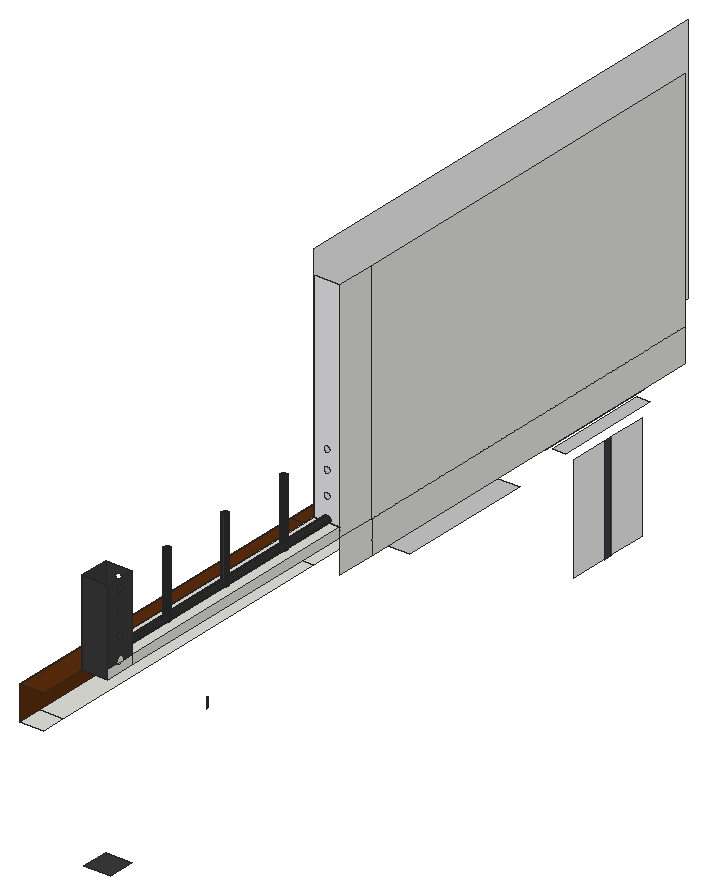
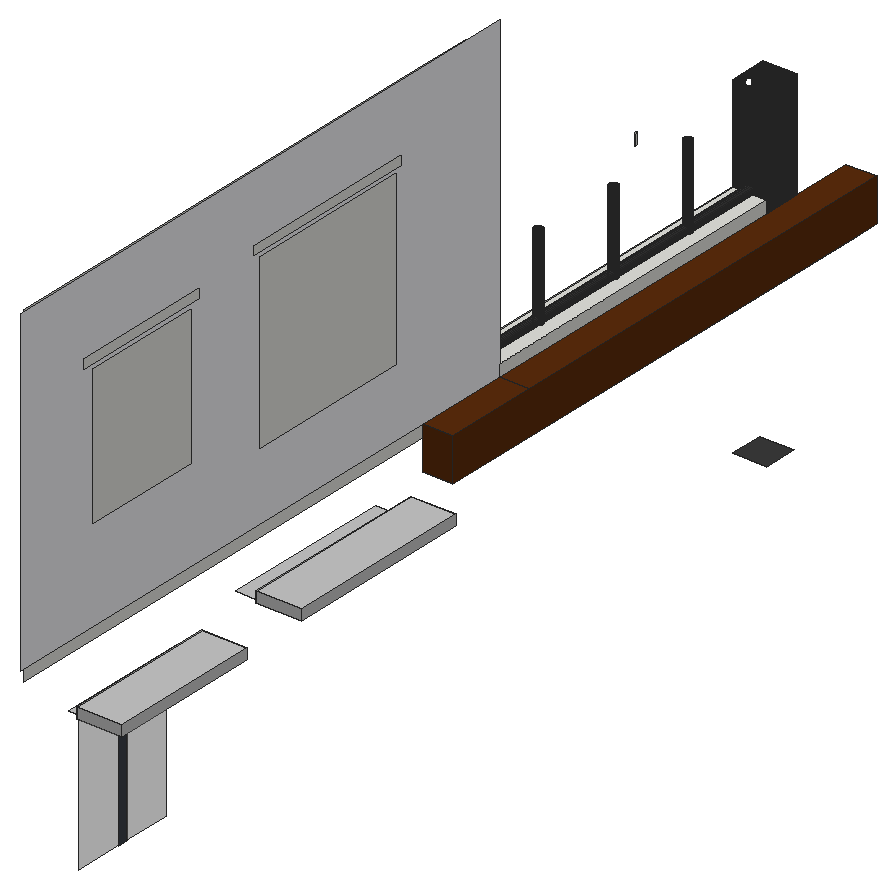
# SketchUp Ruby script. Lengths in inches.
U = 1.inch
M = Sketchup.active_model
def pt(a) = Geom::Point3d.new(a.map { |v| v * U })
def face(e, loops, mat)
  f = e.add_face(loops[0].map { |a| pt(a) })
  loops[1..].each { |l| e.add_face(l.map { |a| pt(a) }).erase! }
  f.material = f.back_material = mat if mat
  f
end
# faces: each face lists its corners as indices into pts; further lists are holes
def faces(e, pts, list, mat = nil) = list.each { |f| face(e, (f[0].is_a?(Array) ? f : [f]).map { |l| l.map { |i| pts[i] } }, mat) }
# xy, xz, yz: faces in a plane at the given z, y or x. An outline is a flat list of corners, or four numbers for a rectangle; further outlines are holes
def ring(l) = l.size == 4 ? [[l[0], l[1]], [l[2], l[1]], [l[2], l[3]], [l[0], l[3]]] : l.each_slice(2).to_a
def flat(e, list, mat, &to3) = list.each { |f| face(e, (f[0].is_a?(Array) ? f : [f]).map { |l| ring(l).map { |u, v| to3.(u, v) } }, mat) }
def xy(e, z, list, mat = nil) = flat(e, list, mat) { |x, y| [x, y, z] }
def xz(e, y, list, mat = nil) = flat(e, list, mat) { |x, z| [x, y, z] }
def yz(e, x, list, mat = nil) = flat(e, list, mat) { |y, z| [x, y, z] }
def lines(e, pts, list) = list.each { |a, b| e.add_line(pt(pts[a]), pt(pts[b])) }
# prism: a flat outline (further loops are holes) pulled along v
def prism(e, loops, v, mat = nil)
  f = face(e, loops, mat); d = Geom::Vector3d.new(v.map { |x| x * U })
  f.pushpull(f.normal.samedirection?(d) ? d.length : -d.length)
end
def box(e, o, s, mat = nil) = prism(e, [[o, [o[0] + s[0], o[1], o[2]], [o[0] + s[0], o[1] + s[1], o[2]], [o[0], o[1] + s[1], o[2]]]], [0, 0, s[2]], mat)
def at(x, y, z, deg = 0) = Geom::Transformation.translation(pt([x, y, z])) * Geom::Transformation.rotation(ORIGIN, Z_AXIS, deg.degrees)
def axes(o, x, y, z) = Geom::Transformation.new([*x, 0, *y, 0, *z, 0, *pt(o).to_a, 1])
def part(name) = M.definitions.add(name)
# library, detail: a bought-in or finely detailed component or shape, given as its bounding box
def library(name, o, s) = part(name).tap { |d| box(d.entities, o, s) }
def detail(e, o, s) = box(e.add_group.entities, o, s)
def put(e, d, t, mat = nil) = e.add_instance(d, t).tap { |i| i.material = mat if mat }
def group(e, t, mat = nil) = e.add_group.tap { |g| g.transformation = t; g.material = mat if mat }.entities
root = M.entities
M.materials.add("[0043_SaddleBrown]").color = [91, 44, 12]
M.materials.add("[Blinds Vertical Pattern]").color = [237, 237, 239]
M.materials.add("[Color M02]").color = [198, 198, 198]
M.materials.add("[Color M07]").color = [58, 58, 58]
M.materials.add("[Formica Laminate Dark]").color = [59, 63, 71]
M.materials.add("[Translucent Glass Gray]").color = [128, 128, 128]
M.materials["[Translucent Glass Gray]"].alpha = 0.5
xy(root,315.4375,[[73.92,405.6875,85.98,418.04]],"[Color M07]")
xy(root,369.09,[[73.92,675.92,79.92,724.73]],"[Color M02]")
xy(root,370.21,[[57.67,672.04,73.92,728.61]],"[Color M02]")
xy(root,370.85,[[73.92,581.05,84.11,644.17]],"[Color M02]")
xy(root,372.15,[[57.67,578.07,73.92,647.71]],"[Color M02]")
xy(root,374.09,[[57.67,672.04,73.92,728.61]],"[Color M02]")
xy(root,376.02,[[57.67,578.07,73.92,647.71]],"[Color M02]")
xy(root,381.625,[[63.07,382.09,73.92,393.34],[63.07,393.34,73.92,538.2],[63.07,538.2,73.92,572.7]])
xy(root,397.0625,[[73.92,404.34,85.98,418.04],[[73.92,418.04,85.98,538.2],[79.95,511.66,80.34,511.71,80.7,511.86,81.01,512.1,81.25,512.41,81.4,512.77,81.45,513.16,81.4,513.55,81.25,513.91,81.01,514.22,80.7,514.46,80.34,514.61,79.95,514.66,79.5625,514.61,79.2,514.46,78.89,514.22,78.65,513.91,78.5,513.55,78.45,513.16,78.5,512.77,78.65,512.41,78.89,512.1,79.2,511.86,79.5625,511.71],[79.95,444.41,80.34,444.46,80.7,444.61,81.01,444.85,81.25,445.16,81.4,445.52,81.45,445.91,81.4,446.3,81.25,446.66,81.01,446.97,80.7,447.21,80.34,447.36,79.95,447.41,79.5625,447.36,79.2,447.21,78.89,446.97,78.65,446.66,78.5,446.3,78.45,445.91,78.5,445.52,78.65,445.16,78.89,444.85,79.2,444.61,79.5625,444.46],[79.95,477.84,80.34,477.9,80.7,478.05,81.01,478.28,81.25,478.59,81.4,478.96,81.45,479.34,81.4,479.73,81.25,480.09,81.01,480.41,80.7,480.64,80.34,480.79,79.95,480.84,79.5625,480.79,79.2,480.64,78.89,480.41,78.65,480.09,78.5,479.73,78.45,479.34,78.5,478.96,78.65,478.59,78.89,478.28,79.2,478.05,79.5625,477.9]],[79.95,444.41,79.5625,444.46,79.2,444.61,78.89,444.85,78.65,445.16,78.5,445.52,78.45,445.91,78.5,446.3,78.65,446.66,78.89,446.97,79.2,447.21,79.5625,447.36,79.95,447.41,80.34,447.36,80.7,447.21,81.01,446.97,81.25,446.66,81.4,446.3,81.45,445.91,81.4,445.52,81.25,445.16,81.01,444.85,80.7,444.61,80.34,444.46],[79.95,477.84,79.5625,477.9,79.2,478.05,78.89,478.28,78.65,478.59,78.5,478.96,78.45,479.34,78.5,479.73,78.65,480.09,78.89,480.41,79.2,480.64,79.5625,480.79,79.95,480.84,80.34,480.79,80.7,480.64,81.01,480.41,81.25,480.09,81.4,479.73,81.45,479.34,81.4,478.96,81.25,478.59,81.01,478.28,80.7,478.05,80.34,477.9],[79.95,511.66,79.5625,511.71,79.2,511.86,78.89,512.1,78.65,512.41,78.5,512.77,78.45,513.16,78.5,513.55,78.65,513.91,78.89,514.22,79.2,514.46,79.5625,514.61,79.95,514.66,80.34,514.61,80.7,514.46,81.01,514.22,81.25,513.91,81.4,513.55,81.45,513.16,81.4,512.77,81.25,512.41,81.01,512.1,80.7,511.86,80.34,511.71]])
xy(root,397.0625,[[63.07,382.09,73.92,538.2],[63.07,538.2,73.92,572.7]],"[0043_SaddleBrown]")
xy(root,401.4375,[[[73.92,418.04,85.98,538.2],[79.95,511.66,79.5625,511.71,79.2,511.86,78.89,512.1,78.65,512.41,78.5,512.77,78.45,513.16,78.5,513.55,78.65,513.91,78.89,514.22,79.2,514.46,79.5625,514.61,79.95,514.66,80.34,514.61,80.7,514.46,81.01,514.22,81.25,513.91,81.4,513.55,81.45,513.16,81.4,512.77,81.25,512.41,81.01,512.1,80.7,511.86,80.34,511.71],[79.95,444.41,79.5625,444.46,79.2,444.61,78.89,444.85,78.65,445.16,78.5,445.52,78.45,445.91,78.5,446.3,78.65,446.66,78.89,446.97,79.2,447.21,79.5625,447.36,79.95,447.41,80.34,447.36,80.7,447.21,81.01,446.97,81.25,446.66,81.4,446.3,81.45,445.91,81.4,445.52,81.25,445.16,81.01,444.85,80.7,444.61,80.34,444.46],[79.95,477.84,79.5625,477.9,79.2,478.05,78.89,478.28,78.65,478.59,78.5,478.96,78.45,479.34,78.5,479.73,78.65,480.09,78.89,480.41,79.2,480.64,79.5625,480.79,79.95,480.84,80.34,480.79,80.7,480.64,81.01,480.41,81.25,480.09,81.4,479.73,81.45,479.34,81.4,478.96,81.25,478.59,81.01,478.28,80.7,478.05,80.34,477.9]]])
xz(root,404.34,[[73.92,397.0625,85.98,436.0625]],"[Color M07]")
xz(root,418.04,[[73.92,397.0625,85.98,397.0625,85.98,401.4375,81.15,401.4375,81.15,401.43,80.81,401.17,80.42,401.01,80,400.95,79.58,401.01,79.18,401.17,78.85,401.43,78.84,401.4375,73.92,401.4375],[80,400.95,80.42,401.01,80.81,401.17,81.15,401.43,81.15,401.4375,78.84,401.4375,78.85,401.43,79.18,401.17,79.58,401.01],[78.84,401.4375,81.15,401.4375,81.4,401.77,81.57,402.16,81.62,402.58,81.57,403,81.4,403.39,81.15,403.73,80.81,403.99,80.42,404.15,80,404.2,79.58,404.15,79.18,403.99,78.85,403.73,78.59,403.39,78.43,403,78.37,402.58,78.43,402.16,78.59,401.77]])
xz(root,418.04,[[[73.92,401.4375,73.92,436.0625,85.98,436.0625,85.98,401.4375,81.15,401.4375,81.4,401.77,81.57,402.16,81.62,402.58,81.57,403,81.4,403.39,81.15,403.73,80.81,403.99,80.42,404.15,80,404.2,79.58,404.15,79.18,403.99,78.85,403.73,78.59,403.39,78.43,403,78.37,402.58,78.43,402.16,78.59,401.77,78.84,401.4375],[80,429.95,80.42,430.01,80.81,430.17,81.15,430.43,81.4,430.77,81.57,431.16,81.62,431.58,81.57,432,81.4,432.39,81.15,432.73,80.81,432.99,80.42,433.15,80,433.2,79.58,433.15,79.18,432.99,78.85,432.73,78.59,432.39,78.43,432,78.37,431.58,78.43,431.16,78.59,430.77,78.85,430.43,79.18,430.17,79.58,430.01],[80,421.33,80.42,421.39,80.81,421.55,81.15,421.81,81.4,422.14,81.57,422.53,81.62,422.95,81.57,423.375,81.4,423.77,81.15,424.1,80.81,424.36,80.42,424.52,80,424.58,79.58,424.52,79.18,424.36,78.85,424.1,78.59,423.77,78.43,423.375,78.37,422.95,78.43,422.53,78.59,422.14,78.85,421.81,79.18,421.55,79.58,421.39],[80,410.64,80.42,410.7,80.81,410.86,81.15,411.12,81.4,411.45,81.57,411.85,81.62,412.27,81.57,412.6875,81.4,413.08,81.15,413.42,80.81,413.67,80.42,413.84,80,413.89,79.58,413.84,79.18,413.67,78.85,413.42,78.59,413.08,78.43,412.6875,78.37,412.27,78.43,411.85,78.59,411.45,78.85,411.12,79.18,410.86,79.58,410.7]]],"[Color M07]")
xz(root,538.2,[[73.92,397.0625,85.98,397.0625,85.98,401.4375,81.15,401.4375,81.15,401.43,80.81,401.17,80.42,401.01,80,400.95,79.58,401.01,79.18,401.17,78.85,401.43,78.84,401.4375,73.92,401.4375],[80,400.95,79.58,401.01,79.18,401.17,78.85,401.43,78.84,401.4375,81.15,401.4375,81.15,401.43,80.81,401.17,80.42,401.01]])
xz(root,538.2,[[[73.92,401.4375,78.84,401.4375,78.59,401.77,78.43,402.16,78.37,402.58,78.43,403,78.59,403.39,78.85,403.73,79.18,403.99,79.58,404.15,80,404.2,80.42,404.15,80.81,403.99,81.15,403.73,81.4,403.39,81.57,403,81.62,402.58,81.57,402.16,81.4,401.77,81.15,401.4375,85.98,401.4375,85.98,501.625,73.92,501.625],[80,410.64,79.58,410.7,79.18,410.86,78.85,411.12,78.59,411.45,78.43,411.85,78.37,412.27,78.43,412.6875,78.59,413.08,78.85,413.42,79.18,413.67,79.58,413.84,80,413.89,80.42,413.84,80.81,413.67,81.15,413.42,81.4,413.08,81.57,412.6875,81.62,412.27,81.57,411.85,81.4,411.45,81.15,411.12,80.81,410.86,80.42,410.7],[80,421.33,79.58,421.39,79.18,421.55,78.85,421.81,78.59,422.14,78.43,422.53,78.37,422.95,78.43,423.375,78.59,423.77,78.85,424.1,79.18,424.36,79.58,424.52,80,424.58,80.42,424.52,80.81,424.36,81.15,424.1,81.4,423.77,81.57,423.375,81.62,422.95,81.57,422.53,81.4,422.14,81.15,421.81,80.81,421.55,80.42,421.39],[80,429.95,79.58,430.01,79.18,430.17,78.85,430.43,78.59,430.77,78.43,431.16,78.37,431.58,78.43,432,78.59,432.39,78.85,432.73,79.18,432.99,79.58,433.15,80,433.2,80.42,433.15,80.81,432.99,81.15,432.73,81.4,432.39,81.57,432,81.62,431.58,81.57,431.16,81.4,430.77,81.15,430.43,80.81,430.17,80.42,430.01]]],"[Blinds Vertical Pattern]")
xz(root,572.7,[[63.07,381.625,73.92,397.0625]],"[0043_SaddleBrown]")
xz(root,578.07,[[57.67,372.15,73.92,376.02]],"[Color M02]")
xz(root,647.71,[[57.67,372.15,73.92,376.02]],"[Color M02]")
xz(root,672.04,[[57.67,370.21,73.92,374.09]],"[Color M02]")
xz(root,728.61,[[57.67,370.21,73.92,374.09]],"[Color M02]")
yz(root,57.67,[[672.04,370.21,728.61,374.09],[578.07,372.15,647.71,376.02]],"[Color M02]")
yz(root,63.07,[[382.09,381.625,572.7,397.0625]],"[0043_SaddleBrown]")
yz(root,73.92,[[672.04,370.21,728.61,374.09],[578.07,372.15,647.71,376.02],[418.04,397.0625,538.2,401.4375]])
yz(root,73.92,[[[538.2,397.0625,753.91,512.25],[584.23,421.07,646.54,483.38],[676.68,429.73,721.56,480.23],[581.95,484.43,649.2,488.12],[672.99,481.56,725.89,485.25]]],"[Blinds Vertical Pattern]")
yz(root,73.92,[[404.34,397.0625,418.04,436.0625]],"[Color M07]")
yz(root,79.92,[[698.31,315.55,702.12,364.63]],"[Formica Laminate Dark]")
yz(root,79.92,[[680.38,315.55,698.31,364.63],[702.12,315.55,720.28,364.63]],"[Translucent Glass Gray]")
yz(root,85.98,[[538.2,381.625,556.28,397.0625],[556.28,381.625,737.09,397.0625],[404.34,397.0625,404.34,401.4375,409.49,401.4375,409.6,401.18,409.875,400.82,410.24,400.54,410.66,400.36,411.11,400.3,411.57,400.36,411.99,400.54,412.35,400.82,412.63,401.18,412.73,401.4375,418.04,401.4375,418.04,397.0625],[418.04,397.0625,538.2,401.4375],[538.2,397.0625,556.28,501.625],
  [556.28,397.0625,737.09,501.625],[411.11,400.3,410.66,400.36,410.24,400.54,409.875,400.82,409.6,401.18,409.49,401.4375,412.73,401.4375,412.63,401.18,412.35,400.82,411.99,400.54,411.57,400.36],[409.49,401.4375,409.42,401.6,409.36,402.05,409.42,402.51,409.6,402.93,409.875,403.29,410.24,403.57,410.66,403.75,411.11,403.8,411.57,403.75,411.99,403.57,412.35,403.29,412.63,402.93,412.8,402.51,412.86,402.05,412.8,401.6,412.73,401.4375]])
yz(root,85.98,[[[404.34,401.4375,409.49,401.4375,409.42,401.6,409.36,402.05,409.42,402.51,409.6,402.93,409.875,403.29,410.24,403.57,410.66,403.75,411.11,403.8,411.57,403.75,411.99,403.57,412.35,403.29,412.63,402.93,412.8,402.51,412.86,402.05,412.8,401.6,412.73,401.4375,418.04,401.4375,418.04,436.0625,404.34,436.0625],[411.11,410.55,410.66,410.61,410.24,410.79,409.875,411.07,409.6,411.43,409.42,411.85,409.36,412.3,409.42,412.76,409.6,413.18,409.875,413.54,410.24,413.82,410.66,414,411.11,414.05,411.57,414,411.99,413.82,412.35,413.54,412.63,413.18,412.8,412.76,412.86,412.3,412.8,411.85,412.63,411.43,412.35,411.07,411.99,410.79,411.57,410.61],[411.11,420.8,410.66,420.86,410.24,421.04,409.875,421.32,409.6,421.68,409.42,422.1,409.36,422.55,409.42,423.01,409.6,423.43,409.875,423.79,410.24,424.07,410.66,424.25,411.11,424.3,411.57,424.25,411.99,424.07,412.35,423.79,412.63,423.43,412.8,423.01,412.86,422.55,412.8,422.1,412.63,421.68,412.35,421.32,411.99,421.04,411.57,420.86],[411.11,429.99,410.66,430.05,410.24,430.23,409.875,430.51,409.6,430.87,409.42,431.29,409.36,431.74,409.42,432.2,409.6,432.62,409.875,432.98,410.24,433.26,410.66,433.43,411.11,433.49,411.57,433.43,411.99,433.26,412.35,432.98,412.63,432.62,412.8,432.2,412.86,431.74,412.8,431.29,412.63,430.87,412.35,430.51,411.99,430.23,411.57,430.05]]],"[Color M07]")
p = [[126.78,410.56,397.0625],[126.84,410.12,397.0625],[126.84,410.12,401.4375],[126.78,410.56,401.4375],[126.84,410.99,397.0625],[126.84,410.99,401.4375],
  [79.5625,444.46,397.0625],[79.95,444.41,397.0625],[79.95,444.41,401.4375],[79.5625,444.46,401.4375],[80.34,444.46,397.0625],[80.34,444.46,401.4375],
  [79.2,444.61,397.0625],[79.2,444.61,401.4375],[80.7,444.61,397.0625],[80.7,444.61,401.4375],[78.89,444.85,397.0625],[78.89,444.85,401.4375],
  [81.01,444.85,397.0625],[81.01,444.85,401.4375],[78.65,445.16,397.0625],[78.65,445.16,401.4375],[81.25,445.16,397.0625],[81.25,445.16,401.4375],
  [78.5,445.52,397.0625],[78.5,445.52,401.4375],[81.4,445.52,397.0625],[81.4,445.52,401.4375],[78.45,445.91,397.0625],[78.45,445.91,401.4375],
  [81.45,445.91,397.0625],[81.45,445.91,401.4375],[78.5,446.3,397.0625],[78.5,446.3,401.4375],[81.4,446.3,397.0625],[81.4,446.3,401.4375],
  [78.65,446.66,397.0625],[78.65,446.66,401.4375],[81.25,446.66,397.0625],[81.25,446.66,401.4375],[78.89,446.97,397.0625],[78.89,446.97,401.4375],
  [81.01,446.97,397.0625],[81.01,446.97,401.4375],[79.2,447.21,397.0625],[79.2,447.21,401.4375],[80.7,447.21,397.0625],[80.7,447.21,401.4375],
  [79.5625,447.36,397.0625],[79.5625,447.36,401.4375],[80.34,447.36,397.0625],[80.34,447.36,401.4375],[79.95,447.41,397.0625],[79.95,447.41,401.4375],
  [79.5625,477.9,397.0625],[79.95,477.84,397.0625],[79.95,477.84,401.4375],[79.5625,477.9,401.4375],[80.34,477.9,397.0625],[80.34,477.9,401.4375],
  [79.2,478.05,397.0625],[79.2,478.05,401.4375],[80.7,478.05,397.0625],[80.7,478.05,401.4375],[78.89,478.28,397.0625],[78.89,478.28,401.4375],
  [81.01,478.28,397.0625],[81.01,478.28,401.4375],[78.65,478.59,397.0625],[78.65,478.59,401.4375],[81.25,478.59,397.0625],[81.25,478.59,401.4375],
  [78.5,478.96,397.0625],[78.5,478.96,401.4375],[81.4,478.96,397.0625],[81.4,478.96,401.4375],[78.45,479.34,397.0625],[78.45,479.34,401.4375],
  [81.45,479.34,397.0625],[81.45,479.34,401.4375],[78.5,479.73,397.0625],[78.5,479.73,401.4375],[81.4,479.73,397.0625],[81.4,479.73,401.4375],
  [78.65,480.09,397.0625],[78.65,480.09,401.4375],[81.25,480.09,397.0625],[81.25,480.09,401.4375],[78.89,480.41,397.0625],[78.89,480.41,401.4375],
  [81.01,480.41,397.0625],[81.01,480.41,401.4375],[79.2,480.64,397.0625],[79.2,480.64,401.4375],[80.7,480.64,397.0625],[80.7,480.64,401.4375],
  [79.5625,480.79,397.0625],[79.5625,480.79,401.4375],[80.34,480.79,397.0625],[80.34,480.79,401.4375],[79.95,480.84,397.0625],[79.95,480.84,401.4375],
  [79.2,511.86,397.0625],[79.5625,511.71,397.0625],[79.5625,511.71,401.4375],[79.2,511.86,401.4375],[79.95,511.66,397.0625],[79.95,511.66,401.4375],
  [80.34,511.71,397.0625],[80.34,511.71,401.4375],[80.7,511.86,397.0625],[80.7,511.86,401.4375],[78.89,512.1,397.0625],[78.89,512.1,401.4375],
  [81.01,512.1,397.0625],[81.01,512.1,401.4375],[78.65,512.41,397.0625],[78.65,512.41,401.4375],[81.25,512.41,397.0625],[81.25,512.41,401.4375],
  [78.5,512.77,397.0625],[78.5,512.77,401.4375],[81.4,512.77,397.0625],[81.4,512.77,401.4375],[78.45,513.16,397.0625],[78.45,513.16,401.4375],
  [81.45,513.16,397.0625],[81.45,513.16,401.4375],[78.5,513.55,397.0625],[78.5,513.55,401.4375],[81.4,513.55,397.0625],[81.4,513.55,401.4375],
  [78.65,513.91,397.0625],[78.65,513.91,401.4375],[81.25,513.91,397.0625],[81.25,513.91,401.4375],[78.89,514.22,397.0625],[78.89,514.22,401.4375],
  [81.01,514.22,397.0625],[81.01,514.22,401.4375],[79.2,514.46,397.0625],[79.2,514.46,401.4375],[80.7,514.46,397.0625],[80.7,514.46,401.4375],
  [79.5625,514.61,397.0625],[79.5625,514.61,401.4375],[80.34,514.61,397.0625],[80.34,514.61,401.4375],[79.95,514.66,397.0625],[79.95,514.66,401.4375],
  [79.58,418.04,401.01],[79.18,418.04,401.17],[79.18,538.2,401.17],[79.58,538.2,401.01],[80,418.04,400.95],[80,538.2,400.95],
  [80.42,418.04,401.01],[80.42,538.2,401.01],[80.81,418.04,401.17],[80.81,538.2,401.17],[78.85,418.04,401.43],[78.85,538.2,401.43],
  [81.15,418.04,401.43],[81.15,538.2,401.43],[78.84,418.04,401.4375],[78.59,418.04,401.77],[78.59,538.2,401.77],[78.84,538.2,401.4375],
  [81.15,418.04,401.4375],[81.15,538.2,401.4375],[81.4,538.2,401.77],[81.4,418.04,401.77],[79.5625,444.46,431.16],[79.95,444.41,431.16],
  [80.34,444.46,431.16],[79.2,444.61,431.16],[80.7,444.61,431.16],[78.89,444.85,431.16],[81.01,444.85,431.16],[78.65,445.16,431.16],
  [81.25,445.16,431.16],[78.5,445.52,431.16],[81.4,445.52,431.16],[78.45,445.91,431.16],[81.45,445.91,431.16],[78.5,446.3,431.16],
  [81.4,446.3,431.16],[78.65,446.66,431.16],[81.25,446.66,431.16],[78.89,446.97,431.16],[81.01,446.97,431.16],[79.2,447.21,431.16],
  [80.7,447.21,431.16],[79.5625,447.36,431.16],[80.34,447.36,431.16],[79.95,447.41,431.16],[79.5625,477.9,431],[79.95,477.84,431],
  [80.34,477.9,431],[79.2,478.05,431],[80.7,478.05,431],[78.89,478.28,431],[81.01,478.28,431],[78.65,478.59,431],
  [81.25,478.59,431],[78.5,478.96,431],[81.4,478.96,431],[78.45,479.34,431],[81.45,479.34,431],[78.5,479.73,431],
  [81.4,479.73,431],[78.65,480.09,431],[81.25,480.09,431],[78.89,480.41,431],[81.01,480.41,431],[79.2,480.64,431],
  [80.7,480.64,431],[79.5625,480.79,431],[80.34,480.79,431],[79.95,480.84,431],[79.2,511.86,431.875],[79.5625,511.71,431.875],
  [79.95,511.66,431.875],[80.34,511.71,431.875],[80.7,511.86,431.875],[78.89,512.1,431.875],[81.01,512.1,431.875],[78.65,512.41,431.875],
  [81.25,512.41,431.875],[78.5,512.77,431.875],[81.4,512.77,431.875],[78.45,513.16,431.875],[81.45,513.16,431.875],[78.5,513.55,431.875],
  [81.4,513.55,431.875],[78.65,513.91,431.875],[81.25,513.91,431.875],[78.89,514.22,431.875],[81.01,514.22,431.875],[79.2,514.46,431.875],
  [80.7,514.46,431.875],[79.5625,514.61,431.875],[80.34,514.61,431.875],[79.95,514.66,431.875],[78.43,418.04,402.16],[78.43,538.2,402.16],
  [81.57,418.04,402.16],[81.57,538.2,402.16],[78.37,418.04,402.58],[78.37,538.2,402.58],[81.62,418.04,402.58],[81.62,538.2,402.58],
  [78.43,418.04,403],[78.43,538.2,403],[81.57,418.04,403],[81.57,538.2,403],[78.59,418.04,403.39],[78.59,538.2,403.39],
  [81.4,418.04,403.39],[81.4,538.2,403.39],[78.85,418.04,403.73],[78.85,538.2,403.73],[81.15,418.04,403.73],[81.15,538.2,403.73],
  [79.18,418.04,403.99],[79.18,538.2,403.99],[80.81,418.04,403.99],[80.81,538.2,403.99],[79.58,418.04,404.15],[79.58,538.2,404.15],
  [80.42,418.04,404.15],[80.42,538.2,404.15],[80,418.04,404.2],[80,538.2,404.2]]
faces(root,p,[[0,1,2,3],[4,0,3,5],[6,7,8,9],[7,10,11,8],[12,6,9,13],[10,14,15,11],[16,12,13,17],[14,18,19,15],
  [20,16,17,21],[18,22,23,19],[24,20,21,25],[22,26,27,23],[28,24,25,29],[26,30,31,27],[32,28,29,33],[30,34,35,31],
  [36,32,33,37],[34,38,39,35],[40,36,37,41],[38,42,43,39],[44,40,41,45],[42,46,47,43],[48,44,45,49],[46,50,51,47],
  [52,48,49,53],[50,52,53,51],[54,55,56,57],[55,58,59,56],[60,54,57,61],[58,62,63,59],[64,60,61,65],[62,66,67,63],
  [68,64,65,69],[66,70,71,67],[72,68,69,73],[70,74,75,71],[76,72,73,77],[74,78,79,75],[80,76,77,81],[78,82,83,79],
  [84,80,81,85],[82,86,87,83],[88,84,85,89],[86,90,91,87],[92,88,89,93],[90,94,95,91],[96,92,93,97],[94,98,99,95],
  [100,96,97,101],[98,100,101,99],[102,103,104,105],[103,106,107,104],[106,108,109,107],[108,110,111,109],[112,102,105,113],[110,114,115,111],
  [116,112,113,117],[114,118,119,115],[120,116,117,121],[118,122,123,119],[124,120,121,125],[122,126,127,123],[128,124,125,129],[126,130,131,127],
  [132,128,129,133],[130,134,135,131],[136,132,133,137],[134,138,139,135],[140,136,137,141],[138,142,143,139],[144,140,141,145],[142,146,147,143],
  [148,144,145,149],[146,148,149,147]])
faces(root,p,[[150,151,152,153],[154,150,153,155],[156,154,155,157],[158,156,157,159],[151,160,161,152],[162,158,159,163],[164,165,166,167,161,160],[168,162,163,169,170,171],
  [172,9,8,173],[173,8,11,174],[175,13,9,172],[174,11,15,176],[177,17,13,175],[176,15,19,178],[179,21,17,177],[178,19,23,180],
  [181,25,21,179],[180,23,27,182],[183,29,25,181],[182,27,31,184],[185,33,29,183],[184,31,35,186],[187,37,33,185],[186,35,39,188],
  [189,41,37,187],[188,39,43,190],[191,45,41,189],[190,43,47,192],[193,49,45,191],[192,47,51,194],[195,53,49,193],[194,51,53,195],
  [196,57,56,197],[197,56,59,198],[199,61,57,196],[198,59,63,200],[201,65,61,199],[200,63,67,202],[203,69,65,201],[202,67,71,204],
  [205,73,69,203],[204,71,75,206],[207,77,73,205],[206,75,79,208],[209,81,77,207],[208,79,83,210],[211,85,81,209],[210,83,87,212],
  [213,89,85,211],[212,87,91,214],[215,93,89,213],[214,91,95,216],[217,97,93,215],[216,95,99,218],[219,101,97,217],[218,99,101,219],
  [220,105,104,221],[221,104,107,222],[222,107,109,223],[223,109,111,224],[225,113,105,220],[224,111,115,226],[227,117,113,225],[226,115,119,228],
  [229,121,117,227],[228,119,123,230],[231,125,121,229],[230,123,127,232],[233,129,125,231],[232,127,131,234],[235,133,129,233],[234,131,135,236],
  [237,137,133,235],[236,135,139,238],[239,141,137,237],[238,139,143,240],[241,145,141,239],[240,143,147,242],[243,149,145,241],[242,147,149,243],
  [165,244,245,166],[246,171,170,247],[244,248,249,245],[250,246,247,251],[248,252,253,249],[254,250,251,255],[252,256,257,253],[258,254,255,259],
  [256,260,261,257],[262,258,259,263],[260,264,265,261],[266,262,263,267],[264,268,269,265],[270,266,267,271],[268,272,273,269],[272,270,271,273]],"[Color M07]")
